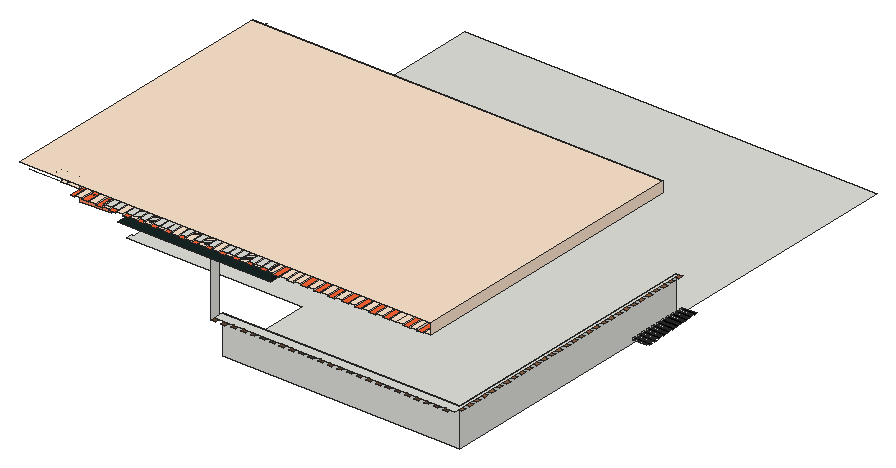
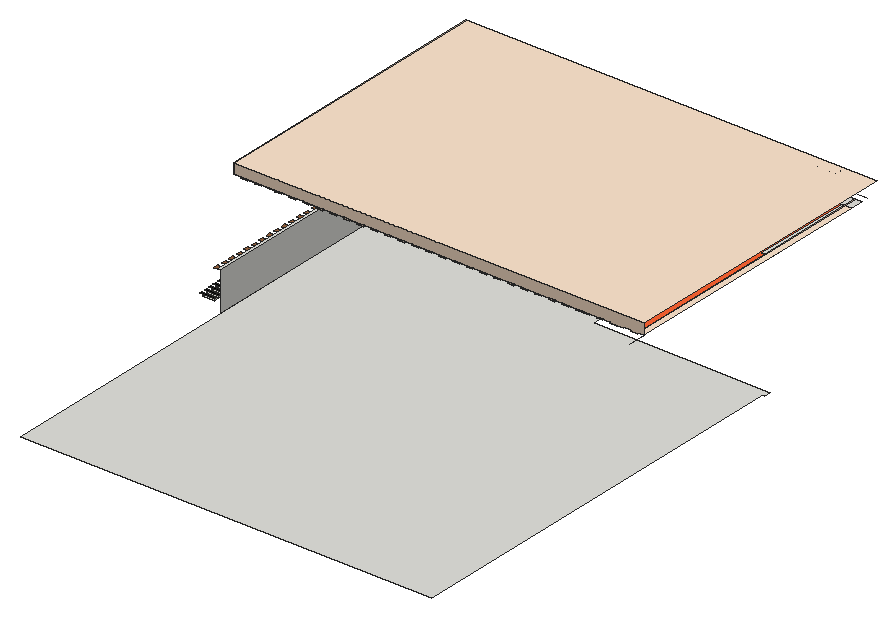
# SketchUp Ruby script. Lengths in inches.
U = 1.inch
M = Sketchup.active_model
def pt(a) = Geom::Point3d.new(a.map { |v| v * U })
def face(e, loops, mat)
  f = e.add_face(loops[0].map { |a| pt(a) })
  loops[1..].each { |l| e.add_face(l.map { |a| pt(a) }).erase! }
  f.material = f.back_material = mat if mat
  f
end
# faces: each face lists its corners as indices into pts; further lists are holes
def faces(e, pts, list, mat = nil) = list.each { |f| face(e, (f[0].is_a?(Array) ? f : [f]).map { |l| l.map { |i| pts[i] } }, mat) }
# xy, xz, yz: faces in a plane at the given z, y or x. An outline is a flat list of corners, or four numbers for a rectangle; further outlines are holes
def ring(l) = l.size == 4 ? [[l[0], l[1]], [l[2], l[1]], [l[2], l[3]], [l[0], l[3]]] : l.each_slice(2).to_a
def flat(e, list, mat, &to3) = list.each { |f| face(e, (f[0].is_a?(Array) ? f : [f]).map { |l| ring(l).map { |u, v| to3.(u, v) } }, mat) }
def xy(e, z, list, mat = nil) = flat(e, list, mat) { |x, y| [x, y, z] }
def xz(e, y, list, mat = nil) = flat(e, list, mat) { |x, z| [x, y, z] }
def yz(e, x, list, mat = nil) = flat(e, list, mat) { |y, z| [x, y, z] }
def lines(e, pts, list) = list.each { |a, b| e.add_line(pt(pts[a]), pt(pts[b])) }
# prism: a flat outline (further loops are holes) pulled along v
def prism(e, loops, v, mat = nil)
  f = face(e, loops, mat); d = Geom::Vector3d.new(v.map { |x| x * U })
  f.pushpull(f.normal.samedirection?(d) ? d.length : -d.length)
end
def box(e, o, s, mat = nil) = prism(e, [[o, [o[0] + s[0], o[1], o[2]], [o[0] + s[0], o[1] + s[1], o[2]], [o[0], o[1] + s[1], o[2]]]], [0, 0, s[2]], mat)
def at(x, y, z, deg = 0) = Geom::Transformation.translation(pt([x, y, z])) * Geom::Transformation.rotation(ORIGIN, Z_AXIS, deg.degrees)
def axes(o, x, y, z) = Geom::Transformation.new([*x, 0, *y, 0, *z, 0, *pt(o).to_a, 1])
def part(name) = M.definitions.add(name)
# library, detail: a bought-in or finely detailed component or shape, given as its bounding box
def library(name, o, s) = part(name).tap { |d| box(d.entities, o, s) }
def detail(e, o, s) = box(e.add_group.entities, o, s)
def put(e, d, t, mat = nil) = e.add_instance(d, t).tap { |i| i.material = mat if mat }
def group(e, t, mat = nil) = e.add_group.tap { |g| g.transformation = t; g.material = mat if mat }.entities
root = M.entities
M.materials.add("B03_Apricot_Glow").color = [255, 140, 101]
M.materials.add("B04_Peach_Ember").color = [255, 101, 50]
M.materials.add("C01_Vanilla_Cream").color = [255, 230, 206]
M.materials.add("M08_Obsidian_Black").color = [23, 37, 38]
M.materials.add("M09_Shadow_Night").color = [0, 0, 0]
M.materials.add("Wood_Veneer_15_1K").color = [150, 100, 65]
M.materials.add("Wood_Veneer_15_1K1").color = [103, 69, 45]
xy(root,519.54,[[222,184.49,443.5,184.49,443.5,671.23,59.5,671.23,59.5,284.23,57.3,284.23,57.3,278.44,222,278.44]])
xy(root,527.89,[[449.91,378.77,463.47,381.22],[449.91,384.31,463.21,386.76],[449.91,389.85,462.95,392.29],[449.91,395.39,462.69,397.83],[449.91,400.92,462.43,403.37],
  [449.91,406.46,462.17,408.91],[449.91,412,461.91,414.45],[449.91,417.54,461.65,419.99],[449.91,423.08,461.39,425.52],[449.91,428.62,461.125,431.0625],
  [449.91,434.15,460.87,436.6]])
xy(root,529.36,[[449.91,378.77,466.08,381.22],[449.91,384.31,465.82,386.76],[449.91,389.85,465.56,392.29],[449.91,395.39,465.3,397.83],[449.91,400.92,465.04,403.37],
  [449.91,406.46,464.78,408.91],[449.91,412,464.51,414.45],[449.91,417.54,464.25,419.99],[449.91,423.08,463.99,425.52],[449.91,428.62,463.73,431.0625],
  [449.91,434.15,463.47,436.6]],"M09_Shadow_Night")
xy(root,555.54,[[222,175.23,446.91,175.23,446.91,436.68,443.5,436.68,443.5,184.49,222,184.49]])
xy(root,555.54,[[446.91,179.58,449.91,183.94],[446.91,188.3,449.91,192.66],[446.91,197.01,449.91,201.37],[446.91,205.73,449.91,210.09],[446.91,214.44,449.91,218.8],
  [446.91,223.16,449.91,227.52],[446.91,231.875,449.91,236.23],[446.91,240.59,449.91,244.95],[446.91,249.31,449.91,253.66],[446.91,258.02,449.91,262.38],
  [446.91,266.74,449.91,271.09],[446.91,275.45,449.91,279.81],[446.91,284.17,449.91,288.52],[446.91,292.88,449.91,297.24],[446.91,301.6,449.91,305.95],
  [446.91,310.3125,449.91,314.67],[446.91,319.03,449.91,323.38],[446.91,327.74,449.91,332.1],[446.91,336.46,449.91,340.82],[446.91,345.17,449.91,349.53],
  [446.91,353.89,449.91,358.25],[446.91,362.6,449.91,366.96],[446.91,371.32,449.91,375.68],[446.91,380.03,449.91,384.39],[446.91,388.75,449.91,393.11],
  [446.91,397.46,449.91,401.82],[446.91,406.18,449.91,410.54],[446.91,414.89,449.91,419.25],[446.91,423.61,449.91,427.97],[446.91,432.33,449.91,436.68]],"Wood_Veneer_15_1K")
xy(root,555.54,[[222,171,226.5,175.23],[231,171,235.49,175.23],[239.99,172.23,244.49,175.23],[248.99,172.23,253.49,175.23],[257.99,172.23,262.48,175.23],
  [266.98,172.23,271.48,175.23],[275.98,172.23,280.48,175.23],[284.97,172.23,289.47,175.23],[293.97,172.23,298.47,175.23],[302.97,172.23,307.47,175.23],
  [311.96,172.23,316.46,175.23],[320.96,172.23,325.46,175.23],[329.96,172.23,334.46,175.23],[338.95,172.23,343.45,175.23],[347.95,172.23,352.45,175.23],
  [356.95,172.23,361.44,175.23],[365.94,172.23,370.44,175.23],[374.9375,172.23,379.4375,175.23],[383.9375,172.23,388.43,175.23],[392.93,172.23,397.43,175.23],
  [401.93,172.23,406.43,175.23],[410.92,172.23,415.42,175.23],[419.92,172.23,424.42,175.23],[428.92,172.23,433.42,175.23],[437.91,172.23,442.41,175.23]],"Wood_Veneer_15_1K1")
xy(root,619.42,[[148.69,154,148.69,171,222,171,222,273.3,291.66,273.3,291.66,154]],"M08_Obsidian_Black")
xy(root,628.54,[[107.56,151,107.56,168,104.71,168,104.71,183.99,111.09,183.99,111.09,151],[117.48,151,123.87,183.99],[130.25,151,136.64,183.99],[143.03,151,149.41,183.99],[155.8,151,162.1875,183.99],
  [168.57,151,174.96,183.99],[181.35,151,187.73,183.99],[194.12,151,200.51,183.99],[206.89,151,213.28,183.99],[219.67,151,226.05,183.99],
  [232.4375,151,238.83,183.99],[245.21,151,251.6,183.99],[257.98,151,264.37,183.99],[270.76,151,277.14,183.99],[283.53,151,289.92,183.99],
  [296.3,151,302.69,183.99],[321.85,151,328.24,183.99],[334.625,151,341.01,183.99],[347.4,151,353.78,183.99],[360.17,151,366.56,183.99],
  [372.94,151,379.33,183.99],[385.72,151,392.1,183.99],[398.49,151,404.88,183.99],[417.65,151,424.04,422.07],[430.42,151,436.81,422.07],
  [66.39,168,72.77,422.07],[79.16,168,85.55,422.07],[85.55,168,91.93,422.07],[104.71,186.99,111.09,386.08],[117.48,186.99,123.87,386.08],
  [130.25,186.99,136.64,386.08],[143.03,186.99,149.41,386.08],[155.8,186.99,162.1875,386.08],[168.57,186.99,174.96,386.08],[181.35,186.99,187.73,386.08],
  [194.12,186.99,200.51,386.08],[206.89,186.99,213.28,386.08],[219.67,186.99,226.05,386.08],[232.4375,186.99,238.83,386.08],[245.21,186.99,251.6,386.08],
  [257.98,186.99,264.37,386.08],[270.76,186.99,277.14,386.08],[283.53,186.99,289.92,386.08],[296.3,186.99,302.69,386.08],[309.08,186.99,315.46,386.08],
  [321.85,186.99,328.24,386.08],[334.625,186.99,341.01,386.08],[347.4,186.99,353.78,386.08],[360.17,186.99,366.56,386.08],[372.94,186.99,379.33,386.08],
  [385.72,186.99,392.1,386.08],[398.49,186.99,404.88,386.08],[98.32,389.08,104.71,422.07],[111.09,389.08,117.48,422.07],[117.48,389.08,123.87,422.07],
  [130.25,389.08,136.64,422.07],[143.03,389.08,149.41,422.07],[155.8,389.08,162.1875,422.07],[168.57,389.08,174.96,422.07],[181.35,389.08,187.73,422.07],
  [194.12,389.08,200.51,422.07],[206.89,389.08,213.28,422.07],[219.67,389.08,226.05,422.07],[232.4375,389.08,238.83,422.07],[245.21,389.08,251.6,422.07],
  [257.98,389.08,264.37,422.07],[270.76,389.08,277.14,422.07],[283.53,389.08,289.92,422.07],[296.3,389.08,302.69,422.07],[309.08,389.08,315.46,422.07],
  [321.85,389.08,328.24,422.07],[334.625,389.08,341.01,422.07],[347.4,389.08,353.78,422.07],[360.17,389.08,366.56,422.07],[372.94,389.08,379.33,422.07],
  [385.72,389.08,392.1,422.07],[398.49,389.08,404.88,422.07]],"B04_Peach_Ember")
xy(root,628.54,[[309.08,151,315.46,183.99]],"C01_Vanilla_Cream")
xy(root,629.54,[[135.55,154,291.66,154,291.66,273.3,222,273.3,222,180,135.55,180],[60,168,89.98,180],[60,180,69,273]])
xy(root,629.54,[[98.32,168,104.71,183.99],[95.99,186.99,98.32,386.08],[98.32,186.99,104.71,386.08]],"B04_Peach_Ember")
xy(root,629.54,[[111.09,151,117.48,183.99],[123.87,151,130.25,183.99],[136.64,151,143.03,183.99],[149.41,151,155.8,183.99],[162.1875,151,168.57,183.99],
  [174.96,151,181.35,183.99],[187.73,151,194.12,183.99],[200.51,151,206.89,183.99],[213.28,151,219.67,183.99],[226.05,151,232.4375,183.99],
  [238.83,151,245.21,183.99],[251.6,151,257.98,183.99],[264.37,151,270.76,183.99],[277.14,151,283.53,183.99],[289.92,151,296.3,183.99],
  [302.69,151,309.08,183.99],[315.46,151,321.85,183.99],[328.24,151,334.625,183.99],[341.01,151,347.4,183.99],[353.78,151,360.17,183.99],
  [366.56,151,372.94,183.99],[379.33,151,385.72,183.99],[392.1,151,398.49,183.99],[404.88,151,404.88,183.99,410.21,183.99,410.21,389.08,404.88,389.08,404.88,422.07,411.26,422.07,411.26,151],[411.26,151,417.65,422.07],
  [424.04,151,430.42,422.07],[436.81,151,443.2,422.07],[89.98,161,95.75,161,96,168,89.98,168],[95.75,161,96,168,107.56,168,107.56,161],[60,168,66.39,422.07],
  [72.77,168,79.16,422.07],[91.93,168,91.93,422.07,98.32,422.07,98.32,389.08,92.99,389.08,92.99,183.99,98.32,183.99,98.32,168],[[92.99,183.99,410.21,389.08],[95.99,186.99,407.21,386.08]],[111.09,186.99,117.48,386.08],[123.87,186.99,130.25,386.08],
  [136.64,186.99,143.03,386.08],[149.41,186.99,155.8,386.08],[162.1875,186.99,168.57,386.08],[174.96,186.99,181.35,386.08],[187.73,186.99,194.12,386.08],
  [200.51,186.99,206.89,386.08],[213.28,186.99,219.67,386.08],[226.05,186.99,232.4375,386.08],[238.83,186.99,245.21,386.08],[251.6,186.99,257.98,386.08],
  [264.37,186.99,270.76,386.08],[277.14,186.99,283.53,386.08],[289.92,186.99,296.3,386.08],[302.69,186.99,309.08,386.08],[315.46,186.99,321.85,386.08],
  [328.24,186.99,334.625,386.08],[341.01,186.99,347.4,386.08],[353.78,186.99,360.17,386.08],[366.56,186.99,372.94,386.08],[379.33,186.99,385.72,386.08],
  [392.1,186.99,398.49,386.08],[404.88,186.99,407.21,386.08],[98.32,389.08,104.71,422.07],[104.71,389.08,111.09,422.07],[111.09,389.08,123.87,422.07],
  [123.87,389.08,130.25,422.07],[130.25,389.08,136.64,422.07],[136.64,389.08,143.03,422.07],[143.03,389.08,149.41,422.07],[149.41,389.08,155.8,422.07],
  [155.8,389.08,162.1875,422.07],[162.1875,389.08,168.57,422.07],[168.57,389.08,174.96,422.07],[174.96,389.08,181.35,422.07],[181.35,389.08,187.73,422.07],
  [187.73,389.08,194.12,422.07],[194.12,389.08,200.51,422.07],[200.51,389.08,206.89,422.07],[206.89,389.08,213.28,422.07],[213.28,389.08,219.67,422.07],
  [219.67,389.08,226.05,422.07],[226.05,389.08,232.4375,422.07],[232.4375,389.08,238.83,422.07],[238.83,389.08,245.21,422.07],[245.21,389.08,251.6,422.07],
  [251.6,389.08,257.98,422.07],[257.98,389.08,264.37,422.07],[264.37,389.08,270.76,422.07],[270.76,389.08,277.14,422.07],[277.14,389.08,283.53,422.07],
  [283.53,389.08,289.92,422.07],[289.92,389.08,296.3,422.07],[296.3,389.08,302.69,422.07],[302.69,389.08,309.08,422.07],[309.08,389.08,315.46,422.07],
  [315.46,389.08,321.85,422.07],[321.85,389.08,328.24,422.07],[328.24,389.08,334.625,422.07],[334.625,389.08,341.01,422.07],[341.01,389.08,347.4,422.07],
  [347.4,389.08,353.78,422.07],[353.78,389.08,360.17,422.07],[360.17,389.08,366.56,422.07],[366.56,389.08,372.94,422.07],[372.94,389.08,379.33,422.07],
  [379.33,389.08,385.72,422.07],[385.72,389.08,392.1,422.07],[392.1,389.08,398.49,422.07],[398.49,389.08,404.88,422.07]],"C01_Vanilla_Cream")
xy(root,639.54,[[60,151,443.2,422.07]],"C01_Vanilla_Cream")
xz(root,168,[[89.98,628.54,91.93,629.54],[104.71,628.54,107.56,629.54]],"C01_Vanilla_Cream")
xz(root,183.99,[[104.71,628.54,111.09,629.54],[117.48,628.54,123.87,629.54],[130.25,628.54,136.64,629.54],[143.03,628.54,149.41,629.54],[155.8,628.54,162.1875,629.54],
  [168.57,628.54,174.96,629.54],[181.35,628.54,187.73,629.54],[194.12,628.54,200.51,629.54],[206.89,628.54,213.28,629.54],[219.67,628.54,226.05,629.54],
  [232.4375,628.54,238.83,629.54],[245.21,628.54,251.6,629.54],[257.98,628.54,264.37,629.54],[270.76,628.54,277.14,629.54],[283.53,628.54,289.92,629.54],
  [296.3,628.54,302.69,629.54],[309.08,628.54,315.46,629.54],[321.85,628.54,328.24,629.54],[334.625,628.54,341.01,629.54],[347.4,628.54,353.78,629.54],
  [360.17,628.54,366.56,629.54],[372.94,628.54,379.33,629.54],[385.72,628.54,392.1,629.54],[398.49,628.54,404.88,629.54]],"C01_Vanilla_Cream")
xz(root,184.49,[[222,519.54,443.5,555.54]])
xz(root,186.99,[[104.71,628.54,111.09,629.54],[117.48,628.54,123.87,629.54],[130.25,628.54,136.64,629.54],[143.03,628.54,149.41,629.54],[155.8,628.54,162.1875,629.54],
  [168.57,628.54,174.96,629.54],[181.35,628.54,187.73,629.54],[194.12,628.54,200.51,629.54],[206.89,628.54,213.28,629.54],[219.67,628.54,226.05,629.54],
  [232.4375,628.54,238.83,629.54],[245.21,628.54,251.6,629.54],[257.98,628.54,264.37,629.54],[270.76,628.54,277.14,629.54],[283.53,628.54,289.92,629.54],
  [296.3,628.54,302.69,629.54],[309.08,628.54,315.46,629.54],[321.85,628.54,328.24,629.54],[334.625,628.54,341.01,629.54],[347.4,628.54,353.78,629.54],
  [360.17,628.54,366.56,629.54],[372.94,628.54,379.33,629.54],[385.72,628.54,392.1,629.54],[398.49,628.54,404.88,629.54]],"C01_Vanilla_Cream")
xz(root,273.3,[[222,619.42,291.66,629.54]],"M08_Obsidian_Black")
xz(root,386.08,[[104.71,628.54,111.09,629.54],[117.48,628.54,123.87,629.54],[130.25,628.54,136.64,629.54],[143.03,628.54,149.41,629.54],[155.8,628.54,162.1875,629.54],
  [168.57,628.54,174.96,629.54],[181.35,628.54,187.73,629.54],[194.12,628.54,200.51,629.54],[206.89,628.54,213.28,629.54],[219.67,628.54,226.05,629.54],
  [232.4375,628.54,238.83,629.54],[245.21,628.54,251.6,629.54],[257.98,628.54,264.37,629.54],[270.76,628.54,277.14,629.54],[283.53,628.54,289.92,629.54],
  [296.3,628.54,302.69,629.54],[309.08,628.54,315.46,629.54],[321.85,628.54,328.24,629.54],[334.625,628.54,341.01,629.54],[347.4,628.54,353.78,629.54],
  [360.17,628.54,366.56,629.54],[372.94,628.54,379.33,629.54],[385.72,628.54,392.1,629.54],[398.49,628.54,404.88,629.54]],"C01_Vanilla_Cream")
xz(root,389.08,[[98.32,628.54,104.71,629.54],[111.09,628.54,117.48,629.54],[117.48,628.54,123.87,629.54],[130.25,628.54,136.64,629.54],[143.03,628.54,149.41,629.54],
  [155.8,628.54,162.1875,629.54],[168.57,628.54,174.96,629.54],[181.35,628.54,187.73,629.54],[194.12,628.54,200.51,629.54],[206.89,628.54,213.28,629.54],
  [219.67,628.54,226.05,629.54],[232.4375,628.54,238.83,629.54],[245.21,628.54,251.6,629.54],[257.98,628.54,264.37,629.54],[270.76,628.54,277.14,629.54],
  [283.53,628.54,289.92,629.54],[296.3,628.54,302.69,629.54],[309.08,628.54,315.46,629.54],[321.85,628.54,328.24,629.54],[334.625,628.54,341.01,629.54],
  [347.4,628.54,353.78,629.54],[360.17,628.54,366.56,629.54],[372.94,628.54,379.33,629.54],[385.72,628.54,392.1,629.54],[398.49,628.54,404.88,629.54]],"C01_Vanilla_Cream")
xz(root,422.07,[[66.39,628.54,66.39,629.54,60,629.54,60,639.54,443.2,639.54,443.2,629.54,91.93,629.54,91.93,628.54,79.16,628.54,79.16,629.54,72.77,629.54,72.77,628.54],[98.32,628.54,104.71,629.54],[111.09,628.54,123.87,629.54],[130.25,628.54,136.64,629.54],[143.03,628.54,149.41,629.54],
  [155.8,628.54,162.1875,629.54],[168.57,628.54,174.96,629.54],[181.35,628.54,187.73,629.54],[194.12,628.54,200.51,629.54],[206.89,628.54,213.28,629.54],
  [219.67,628.54,226.05,629.54],[232.4375,628.54,238.83,629.54],[245.21,628.54,251.6,629.54],[257.98,628.54,264.37,629.54],[270.76,628.54,277.14,629.54],
  [283.53,628.54,289.92,629.54],[296.3,628.54,302.69,629.54],[309.08,628.54,315.46,629.54],[321.85,628.54,328.24,629.54],[334.625,628.54,341.01,629.54],
  [347.4,628.54,353.78,629.54],[360.17,628.54,366.56,629.54],[372.94,628.54,379.33,629.54],[385.72,628.54,392.1,629.54],[398.49,628.54,404.88,629.54],
  [417.65,628.54,424.04,629.54],[430.42,628.54,436.81,629.54]],"C01_Vanilla_Cream")
yz(root,66.39,[[168,628.54,422.07,629.54]],"C01_Vanilla_Cream")
yz(root,72.77,[[168,628.54,422.07,629.54]],"C01_Vanilla_Cream")
yz(root,79.16,[[168,628.54,422.07,629.54]],"C01_Vanilla_Cream")
yz(root,91.93,[[168,628.54,422.07,629.54]],"C01_Vanilla_Cream")
yz(root,98.32,[[389.08,628.54,422.07,629.54]],"C01_Vanilla_Cream")
yz(root,104.71,[[168,628.54,183.99,629.54],[186.99,628.54,386.08,629.54],[389.08,628.54,422.07,629.54]],"C01_Vanilla_Cream")
yz(root,107.56,[[161,628.54,168,629.54]],"C01_Vanilla_Cream")
yz(root,111.09,[[151,628.54,165.73,629.54],[165.73,628.54,183.99,629.54],[186.99,628.54,386.08,629.54],[389.08,628.54,422.07,629.54]],"C01_Vanilla_Cream")
yz(root,117.48,[[151,628.54,165.45,629.54],[165.45,628.54,183.99,629.54],[186.99,628.54,386.08,629.54]],"C01_Vanilla_Cream")
yz(root,123.87,[[151,628.54,165.17,629.54],[165.17,628.54,183.99,629.54],[186.99,628.54,386.08,629.54],[389.08,628.54,422.07,629.54]],"C01_Vanilla_Cream")
yz(root,130.25,[[151,628.54,164.88,629.54],[164.88,628.54,183.99,629.54],[186.99,628.54,386.08,629.54],[389.08,628.54,422.07,629.54]],"C01_Vanilla_Cream")
yz(root,136.64,[[151,628.54,164.6,629.54],[164.6,628.54,183.99,629.54],[186.99,628.54,386.08,629.54],[389.08,628.54,422.07,629.54]],"C01_Vanilla_Cream")
yz(root,143.03,[[151,628.54,164.32,629.54],[164.32,628.54,183.99,629.54],[186.99,628.54,386.08,629.54],[389.08,628.54,422.07,629.54]],"C01_Vanilla_Cream")
yz(root,149.41,[[151,628.54,164.03,629.54],[164.03,628.54,183.99,629.54],[186.99,628.54,386.08,629.54],[389.08,628.54,422.07,629.54]],"C01_Vanilla_Cream")
yz(root,155.8,[[151,628.54,163.75,629.54],[163.75,628.54,183.99,629.54],[186.99,628.54,386.08,629.54],[389.08,628.54,422.07,629.54]],"C01_Vanilla_Cream")
yz(root,162.1875,[[151,628.54,163.47,629.54],[163.47,628.54,183.99,629.54],[186.99,628.54,386.08,629.54],[389.08,628.54,422.07,629.54]],"C01_Vanilla_Cream")
yz(root,168.57,[[151,628.54,163.18,629.54],[163.18,628.54,183.99,629.54],[186.99,628.54,386.08,629.54],[389.08,628.54,422.07,629.54]],"C01_Vanilla_Cream")
yz(root,174.96,[[151,628.54,162.9,629.54],[162.9,628.54,183.99,629.54],[186.99,628.54,386.08,629.54],[389.08,628.54,422.07,629.54]],"C01_Vanilla_Cream")
yz(root,181.35,[[151,628.54,162.62,629.54],[162.62,628.54,183.99,629.54],[186.99,628.54,386.08,629.54],[389.08,628.54,422.07,629.54]],"C01_Vanilla_Cream")
yz(root,187.73,[[151,628.54,162.33,629.54],[162.33,628.54,183.99,629.54],[186.99,628.54,386.08,629.54],[389.08,628.54,422.07,629.54]],"C01_Vanilla_Cream")
yz(root,194.12,[[151,628.54,162.05,629.54],[162.05,628.54,183.99,629.54],[186.99,628.54,386.08,629.54],[389.08,628.54,422.07,629.54]],"C01_Vanilla_Cream")
yz(root,200.51,[[151,628.54,161.77,629.54],[161.77,628.54,183.99,629.54],[186.99,628.54,386.08,629.54],[389.08,628.54,422.07,629.54]],"C01_Vanilla_Cream")
yz(root,206.89,[[151,628.54,161.48,629.54],[161.48,628.54,183.99,629.54],[186.99,628.54,386.08,629.54],[389.08,628.54,422.07,629.54]],"C01_Vanilla_Cream")
yz(root,213.28,[[151,628.54,161.2,629.54],[161.2,628.54,183.99,629.54],[186.99,628.54,386.08,629.54],[389.08,628.54,422.07,629.54]],"C01_Vanilla_Cream")
yz(root,219.67,[[151,628.54,151.92,629.54],[151.92,628.54,160.92,629.54],[160.92,628.54,183.99,629.54],[186.99,628.54,386.08,629.54],[389.08,628.54,422.07,629.54]],"C01_Vanilla_Cream")
yz(root,222,[[171,555.54,180,619.42]])
yz(root,222,[[180,619.42,273.3,629.54]],"M08_Obsidian_Black")
yz(root,226.05,[[151,628.54,160.63,629.54],[160.63,628.54,183.99,629.54],[186.99,628.54,386.08,629.54],[389.08,628.54,422.07,629.54]],"C01_Vanilla_Cream")
yz(root,232.4375,[[151,628.54,160.35,629.54],[160.35,628.54,183.99,629.54],[186.99,628.54,386.08,629.54],[389.08,628.54,422.07,629.54]],"C01_Vanilla_Cream")
yz(root,238.83,[[151,628.54,160.07,629.54],[160.07,628.54,183.99,629.54],[186.99,628.54,386.08,629.54],[389.08,628.54,422.07,629.54]],"C01_Vanilla_Cream")
yz(root,245.21,[[151,628.54,159.78,629.54],[159.78,628.54,167.2,629.54],[167.2,628.54,183.99,629.54],[186.99,628.54,386.08,629.54],[389.08,628.54,422.07,629.54]],"C01_Vanilla_Cream")
yz(root,251.6,[[151,628.54,159.5,629.54],[159.5,628.54,183.99,629.54],[186.99,628.54,386.08,629.54],[389.08,628.54,422.07,629.54]],"C01_Vanilla_Cream")
yz(root,257.98,[[151,628.54,159.22,629.54],[159.22,628.54,183.99,629.54],[186.99,628.54,386.08,629.54],[389.08,628.54,422.07,629.54]],"C01_Vanilla_Cream")
yz(root,264.37,[[151,628.54,158.93,629.54],[158.93,628.54,183.99,629.54],[186.99,628.54,386.08,629.54],[389.08,628.54,422.07,629.54]],"C01_Vanilla_Cream")
yz(root,270.76,[[151,628.54,158.65,629.54],[158.65,628.54,183.99,629.54],[186.99,628.54,386.08,629.54],[389.08,628.54,422.07,629.54]],"C01_Vanilla_Cream")
yz(root,277.14,[[151,628.54,158.37,629.54],[158.37,628.54,183.99,629.54],[186.99,628.54,386.08,629.54],[389.08,628.54,422.07,629.54]],"C01_Vanilla_Cream")
yz(root,283.53,[[151,628.54,158.08,629.54],[158.08,628.54,183.99,629.54],[186.99,628.54,386.08,629.54],[389.08,628.54,422.07,629.54]],"C01_Vanilla_Cream")
yz(root,289.92,[[151,628.54,157.8,629.54],[157.8,628.54,183.99,629.54],[186.99,628.54,386.08,629.54],[389.08,628.54,422.07,629.54]],"C01_Vanilla_Cream")
yz(root,291.66,[[154,619.42,273.3,629.54]],"M08_Obsidian_Black")
yz(root,296.3,[[151,628.54,157.52,629.54],[157.52,628.54,183.99,629.54],[186.99,628.54,386.08,629.54],[389.08,628.54,422.07,629.54]],"C01_Vanilla_Cream")
yz(root,302.69,[[151,628.54,157.23,629.54],[157.23,628.54,183.99,629.54],[186.99,628.54,386.08,629.54],[389.08,628.54,422.07,629.54]],"C01_Vanilla_Cream")
yz(root,309.08,[[151,628.54,156.95,629.54],[156.95,628.54,157.52,629.54],[157.52,628.54,183.99,629.54],[186.99,628.54,386.08,629.54],[389.08,628.54,422.07,629.54]],"C01_Vanilla_Cream")
yz(root,315.46,[[151,628.54,156.67,629.54],[156.67,628.54,183.99,629.54],[186.99,628.54,386.08,629.54],[389.08,628.54,422.07,629.54]],"C01_Vanilla_Cream")
yz(root,321.85,[[151,628.54,156.38,629.54],[156.38,628.54,183.99,629.54],[186.99,628.54,386.08,629.54],[389.08,628.54,422.07,629.54]],"C01_Vanilla_Cream")
yz(root,328.24,[[151,628.54,156.1,629.54],[156.1,628.54,183.99,629.54],[186.99,628.54,386.08,629.54],[389.08,628.54,422.07,629.54]],"C01_Vanilla_Cream")
yz(root,334.625,[[151,628.54,155.82,629.54],[155.82,628.54,183.99,629.54],[186.99,628.54,386.08,629.54],[389.08,628.54,422.07,629.54]],"C01_Vanilla_Cream")
yz(root,341.01,[[151,628.54,155.53,629.54],[155.53,628.54,156.38,629.54],[156.38,628.54,183.99,629.54],[186.99,628.54,386.08,629.54],[389.08,628.54,422.07,629.54]],"C01_Vanilla_Cream")
yz(root,347.4,[[151,628.54,155.25,629.54],[155.25,628.54,183.99,629.54],[186.99,628.54,386.08,629.54],[389.08,628.54,422.07,629.54]],"C01_Vanilla_Cream")
yz(root,353.78,[[151,628.54,154.97,629.54],[154.97,628.54,156.38,629.54],[156.38,628.54,183.99,629.54],[186.99,628.54,386.08,629.54],[389.08,628.54,422.07,629.54]],"C01_Vanilla_Cream")
yz(root,360.17,[[151,628.54,154.68,629.54],[154.68,628.54,183.99,629.54],[186.99,628.54,386.08,629.54],[389.08,628.54,422.07,629.54]],"C01_Vanilla_Cream")
yz(root,366.56,[[151,628.54,154.4,629.54],[154.4,628.54,183.99,629.54],[186.99,628.54,386.08,629.54],[389.08,628.54,422.07,629.54]],"C01_Vanilla_Cream")
yz(root,372.94,[[151,628.54,154.12,629.54],[154.12,628.54,154.4,629.54],[154.4,628.54,183.99,629.54],[186.99,628.54,386.08,629.54],[389.08,628.54,422.07,629.54]],"C01_Vanilla_Cream")
yz(root,379.33,[[151,628.54,153.83,629.54],[153.83,628.54,183.99,629.54],[186.99,628.54,386.08,629.54],[389.08,628.54,422.07,629.54]],"C01_Vanilla_Cream")
yz(root,385.72,[[151,628.54,153.55,629.54],[153.55,628.54,183.99,629.54],[186.99,628.54,386.08,629.54],[389.08,628.54,422.07,629.54]],"C01_Vanilla_Cream")
yz(root,392.1,[[151,628.54,153.27,629.54],[153.27,628.54,183.99,629.54],[186.99,628.54,386.08,629.54],[389.08,628.54,422.07,629.54]],"C01_Vanilla_Cream")
yz(root,398.49,[[151,628.54,152.98,629.54],[152.98,628.54,183.99,629.54],[186.99,628.54,386.08,629.54],[389.08,628.54,422.07,629.54]],"C01_Vanilla_Cream")
yz(root,404.88,[[151,628.54,152.7,629.54],[152.7,628.54,183.99,629.54],[186.99,628.54,386.08,629.54],[389.08,628.54,422.07,629.54]],"C01_Vanilla_Cream")
yz(root,417.65,[[151,628.54,152.13,629.54],[152.13,628.54,422.07,629.54]],"C01_Vanilla_Cream")
yz(root,424.04,[[151,628.54,151.85,629.54],[151.85,628.54,422.07,629.54]],"C01_Vanilla_Cream")
yz(root,430.42,[[151,628.54,151.57,629.54],[151.57,628.54,422.07,629.54]],"C01_Vanilla_Cream")
yz(root,436.81,[[151,628.54,151.28,629.54],[151.28,628.54,422.07,629.54]],"C01_Vanilla_Cream")
yz(root,443.2,[[151,629.54,422.07,639.54]],"C01_Vanilla_Cream")
yz(root,443.5,[[184.49,519.54,436.68,555.54]])
yz(root,449.91,[[378.77,527.89,381.22,529.36],[384.31,527.89,386.76,529.36],[389.85,527.89,392.29,529.36],[395.39,527.89,397.83,529.36],[400.92,527.89,403.37,529.36],
  [406.46,527.89,408.91,529.36],[412,527.89,414.45,529.36],[417.54,527.89,419.99,529.36],[423.08,527.89,425.52,529.36],[428.62,527.89,431.0625,529.36],
  [434.15,527.89,436.6,529.36]])
p = [[107.56,161,628.54],[107.56,161,618.67],[135.55,162.92,618.67],[135.55,162.92,628.54],[89.98,156,639.54],[89.98,156,639.71],
  [60,161,629.54],[89.98,161,629.54],[95.75,161,629.54],[95.75,161,639.54],[107.56,161,629.54],[107.56,161,639.54],
  [89.98,161,639.54],[436.81,422.07,629.54],[436.81,422.35,629.54],[104.71,166.02,629.54],[104.71,168,629.54],[98.32,166.3,629.54],
  [98.32,168,629.54],[91.93,166.58,629.54],[91.93,168,629.54],[85.55,166.87,629.54],[85.55,168,629.54],[79.16,167.15,629.54],
  [79.16,168,629.54],[72.77,167.43,629.54],[72.77,168,629.54],[66.39,167.72,629.54],[66.39,168,629.54],[60,422.07,629.54],
  [60,439.07,629.54]]
faces(root,p,[[0,1,2,3]],"B03_Apricot_Glow")
lines(root,p,[[4,5],[6,7],[8,9],[10,11],[7,12],[13,14],[15,16],[17,18],[19,20],[21,22],[23,24],[25,26],
  [27,28],[29,30]])
